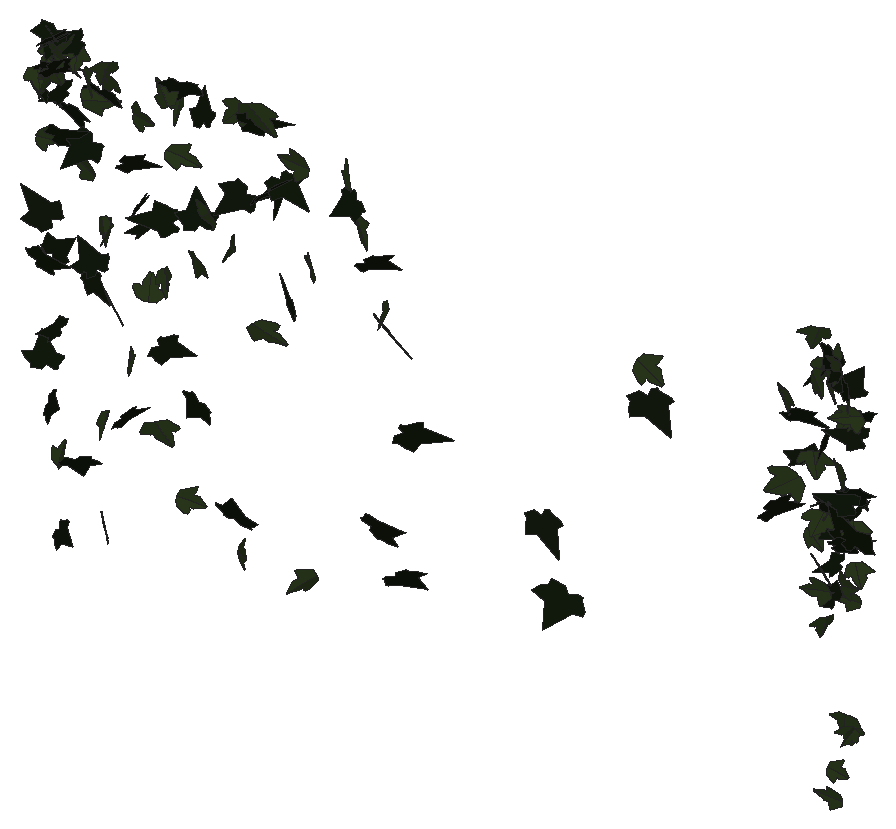
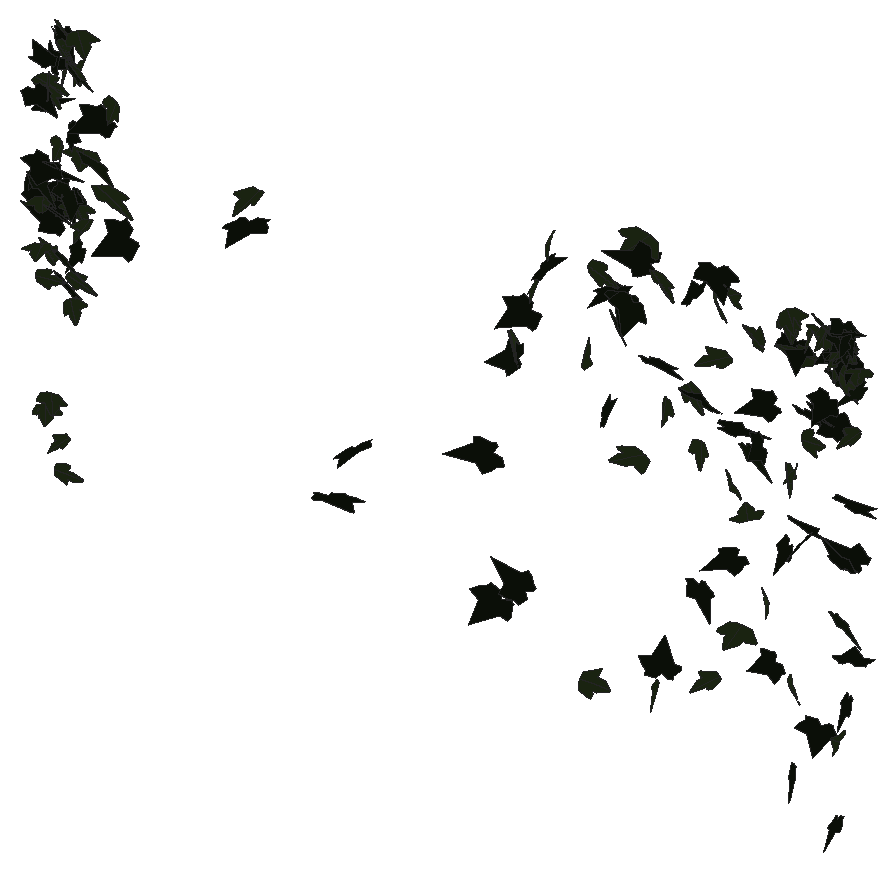
# SketchUp Ruby script. Lengths in inches.
U = 1.inch
M = Sketchup.active_model
def pt(a) = Geom::Point3d.new(a.map { |v| v * U })
def face(e, loops, mat)
  f = e.add_face(loops[0].map { |a| pt(a) })
  loops[1..].each { |l| e.add_face(l.map { |a| pt(a) }).erase! }
  f.material = f.back_material = mat if mat
  f
end
# faces: each face lists its corners as indices into pts; further lists are holes
def faces(e, pts, list, mat = nil) = list.each { |f| face(e, (f[0].is_a?(Array) ? f : [f]).map { |l| l.map { |i| pts[i] } }, mat) }
# xy, xz, yz: faces in a plane at the given z, y or x. An outline is a flat list of corners, or four numbers for a rectangle; further outlines are holes
def ring(l) = l.size == 4 ? [[l[0], l[1]], [l[2], l[1]], [l[2], l[3]], [l[0], l[3]]] : l.each_slice(2).to_a
def flat(e, list, mat, &to3) = list.each { |f| face(e, (f[0].is_a?(Array) ? f : [f]).map { |l| ring(l).map { |u, v| to3.(u, v) } }, mat) }
def xy(e, z, list, mat = nil) = flat(e, list, mat) { |x, y| [x, y, z] }
def xz(e, y, list, mat = nil) = flat(e, list, mat) { |x, z| [x, y, z] }
def yz(e, x, list, mat = nil) = flat(e, list, mat) { |y, z| [x, y, z] }
def lines(e, pts, list) = list.each { |a, b| e.add_line(pt(pts[a]), pt(pts[b])) }
# prism: a flat outline (further loops are holes) pulled along v
def prism(e, loops, v, mat = nil)
  f = face(e, loops, mat); d = Geom::Vector3d.new(v.map { |x| x * U })
  f.pushpull(f.normal.samedirection?(d) ? d.length : -d.length)
end
def box(e, o, s, mat = nil) = prism(e, [[o, [o[0] + s[0], o[1], o[2]], [o[0] + s[0], o[1] + s[1], o[2]], [o[0], o[1] + s[1], o[2]]]], [0, 0, s[2]], mat)
def at(x, y, z, deg = 0) = Geom::Transformation.translation(pt([x, y, z])) * Geom::Transformation.rotation(ORIGIN, Z_AXIS, deg.degrees)
def axes(o, x, y, z) = Geom::Transformation.new([*x, 0, *y, 0, *z, 0, *pt(o).to_a, 1])
def part(name) = M.definitions.add(name)
# library, detail: a bought-in or finely detailed component or shape, given as its bounding box
def library(name, o, s) = part(name).tap { |d| box(d.entities, o, s) }
def detail(e, o, s) = box(e.add_group.entities, o, s)
def put(e, d, t, mat = nil) = e.add_instance(d, t).tap { |i| i.material = mat if mat }
def group(e, t, mat = nil) = e.add_group.tap { |g| g.transformation = t; g.material = mat if mat }.entities
root = M.entities
M.materials.add("1026 AP 7946 SUNNY SIDE UP").color = [254, 231, 186]
M.materials.add("efeu1").color = [18, 25, 13]
M.materials.add("efeu2").color = [43, 57, 29]
c1 = part("ivyleaf_9")
p = [[1.54,2.16,1.25],[1.36,2.04,1.19],[-0.21,0.99,0.68],[-0.71,1.11,0.82],[-0.85,0.86,0.67],[-0.8,0.17,0.21],
  [-0.9,-0.01,0.1],[-0.67,-0.16,-0.02],[-0.08,-0.08,-0.05],[-0.03,-0.6,-0.4],[0.65,-0.88,-0.66],[0.83,-0.6,-0.49],
  [1.29,-0.42,-0.43],[1.8125,-0.07,-0.26],[1.21,0.44,0.15]]
faces(c1.entities,p,[[0,1,2,3,4,5,6,7,8,9,10,11,12,13,14]],"efeu1")
c2 = part("ivyleaf_10")
p = [[0,0.5,-0.03],[-0.0625,2.02,-0.43],[-0.19,2.01,-0.46],[-0.54,1.05,-0.29],[-0.52,0.625,-0.18],[-0.83,0.76,-0.28],
  [-1.16,0.64,-0.33],[-1.15,0.33,-0.24],[-0.77,-0.39,0.02],[-0.3,-0.51,0.16],[0.04,-0.48,0.23],[-0.02,2.01,-0.4375],
  [-0.06,2.01,-0.43],[0.04,-0.49,0.23],[0.67,-0.49,0.14],[1.38,0.36,-0.2],[1.375,0.51,-0.24],[0.81,0.65,-0.19],
  [0.62,0.59,-0.15],[0.6,1.09,-0.28],[0.5,1.23,-0.31]]
faces(c2.entities,p,[[0,1,2,3,4,5,6,7,8,9,10],[11,12,0,13,14,15,16,17,18,19,20]],"efeu2")
put(root,c1,axes([117.92,212.64,266.27],[0.34447,-0.10221,-0.11424],[-0.10357,0.11002,-0.23912],[0.21258,0.21922,0.06863]),"1026 AP 7946 SUNNY SIDE UP")
put(root,c1,axes([118.2,212.71,258.34],[-0.36248,-0.06396,0.109],[0.15543,0.04038,0.24641],[-0.11757,0.25057,-0.01029]),"1026 AP 7946 SUNNY SIDE UP")
put(root,c2,axes([118.03,212.6,266.67],[0.26881,0.19626,0.00102],[0.01701,-0.00958,-0.26778],[-0.30813,0.17069,-0.01389]),"1026 AP 7946 SUNNY SIDE UP")
put(root,c1,axes([118.48,212.51,262.68],[-0.44152,-0.06357,-0.11525],[-0.18136,0.00727,0.29498],[-0.08856,0.30203,-0.02951]),"1026 AP 7946 SUNNY SIDE UP")
put(root,c2,axes([118.14,212.62,264.84],[0.01266,0.11269,0.23888],[0.00793,0.23124,-0.11493],[-0.40441,0.00806,0.00522]),"1026 AP 7946 SUNNY SIDE UP")
put(root,c1,axes([118.29,212.72,257.18],[0.05293,-0.0259,-0.29049],[-0.3113,0.20067,-0.04218],[0.31802,0.20074,0.00706]),"1026 AP 7946 SUNNY SIDE UP")
put(root,c2,axes([118.32,212.88,267.27],[0.23133,0.15211,-0.15112],[-0.14124,-0.11794,-0.2182],[-0.30182,0.17178,-0.01372]),"1026 AP 7946 SUNNY SIDE UP")
put(root,c2,axes([118.28,212.85,266.58],[0.05975,-0.23156,0.20577],[0.06281,-0.19713,-0.24282],[0.4781,0.05484,0.00619]),"1026 AP 7946 SUNNY SIDE UP")
put(root,c1,axes([118.08,213.03,267.7],[0.29837,-0.17045,0.00968],[-0.01091,-0.02317,-0.26194],[0.2683,0.18862,-0.02141]),"1026 AP 7946 SUNNY SIDE UP")
put(root,c1,axes([118.13,213.09,261.29],[-0.13636,0.13153,0.21387],[0.22426,-0.15138,0.15988],[0.31349,0.16551,-0.02134]),"1026 AP 7946 SUNNY SIDE UP")
put(root,c1,axes([117.99,212.66,261.23],[0.09601,-0.03822,0.25968],[0.32127,-0.14806,-0.07492],[0.24033,0.2132,-0.00359]),"1026 AP 7946 SUNNY SIDE UP")
put(root,c1,axes([118.45,212.75,267.66],[0.02147,0.25653,0.0187],[-0.01192,0.01711,-0.2644],[-0.40404,0.01313,0.0088]),"1026 AP 7946 SUNNY SIDE UP")
put(root,c1,axes([118.33,212.92,267.79],[-0.23433,-0.21118,-0.0017],[0.03878,-0.01686,-0.26458],[0.32978,-0.14807,0.0299]),"1026 AP 7946 SUNNY SIDE UP")
put(root,c1,axes([118.49,212.61,267.84],[-0.0099,0.25599,-0.03036],[0.00018,-0.03093,-0.26398],[-0.40545,-0.00627,0.00062]),"1026 AP 7946 SUNNY SIDE UP")
put(root,c2,axes([118.34,212.91,267.35],[-0.08937,0.25025,-0.01074],[-0.00659,-0.01309,-0.26436],[-0.39389,-0.05656,0.00686]),"1026 AP 7946 SUNNY SIDE UP")
put(root,c1,axes([118.62,212.71,259.44],[-0.23134,0.21492,0.03365],[-0.04737,0.01742,-0.26778],[-0.33824,-0.14944,0.01449]),"1026 AP 7946 SUNNY SIDE UP")
put(root,c1,axes([118.47,212.64,267.02],[0.21167,0.214,-0.09142],[-0.05465,-0.08423,-0.26051],[-0.3609,0.13827,-0.01417]),"1026 AP 7946 SUNNY SIDE UP")
put(root,c2,axes([118.73,212.51,267.39],[0.03224,-0.0236,-0.2805],[-0.31872,0.18164,-0.0309],[0.28795,0.20369,-0.0028]),"1026 AP 7946 SUNNY SIDE UP")
put(root,c2,axes([118.45,212.69,266.86],[-0.20915,-0.21356,-0.11347],[0.13001,0.07607,-0.2572],[0.35384,-0.15418,0.02743]),"1026 AP 7946 SUNNY SIDE UP")
put(root,c1,axes([118.26,212.88,267.28],[0.2693,-0.19309,-0.00503],[0.06195,0.03988,-0.25934],[0.29728,0.1666,0.0586]),"1026 AP 7946 SUNNY SIDE UP")
put(root,c1,axes([118.59,212.78,253.63],[0.098,-0.10726,-0.25094],[-0.24061,0.18949,-0.1255],[0.34134,0.16436,-0.01642]),"1026 AP 7946 SUNNY SIDE UP")
put(root,c1,axes([118.83,212.6875,266.38],[-0.2985,0.17637,-0.00799],[-0.01055,-0.02004,-0.26632],[-0.27746,-0.18898,0.01871]),"1026 AP 7946 SUNNY SIDE UP")
put(root,c2,axes([118.7,212.9,267.56],[-0.05796,-0.25516,0.02452],[0.01005,-0.02641,-0.26555],[0.40305,-0.03603,0.01015]),"1026 AP 7946 SUNNY SIDE UP")
put(root,c2,axes([118.71,212.54,255.78],[0.0181,0.14274,-0.22667],[0.0407,0.21936,0.14874],[0.41145,-0.02798,-0.00474]),"1026 AP 7946 SUNNY SIDE UP")
put(root,c1,axes([118.61,212.36,267.09],[0.2386,0.18431,0.18808],[0.20633,0.12653,-0.24461],[-0.35056,0.19992,-0.01596]),"1026 AP 7946 SUNNY SIDE UP")
put(root,c1,axes([118.5,212.73,264.95],[0.3529,0.092,-0.10758],[0.10626,0.10225,0.24182],[0.19201,-0.22567,0.06389]),"1026 AP 7946 SUNNY SIDE UP")
put(root,c1,axes([118.74,212.95,265.76],[0.38897,0.00534,-0.08902],[-0.13488,-0.021,-0.25435],[-0.0188,0.2612,-0.01709]),"1026 AP 7946 SUNNY SIDE UP")
put(root,c2,axes([118.83,212.89,267.68],[-0.09661,-0.19451,-0.1674],[0.11101,0.14627,-0.20845],[0.3816,-0.0918,0.01826]),"1026 AP 7946 SUNNY SIDE UP")
put(root,c1,axes([119.16,212.8125,267.86],[-0.35541,0.12461,-0.0421],[0.04217,-0.03722,-0.26536],[-0.2022,-0.22679,0.01866]),"1026 AP 7946 SUNNY SIDE UP")
put(root,c2,axes([119.04,212.82,267.55],[0.39368,-0.02427,0.06501],[0.09332,-0.03811,-0.25736],[0.05134,0.2554,-0.03068]),"1026 AP 7946 SUNNY SIDE UP")
put(root,c2,axes([119.53,212.78,264.26],[-0.1002,0.04016,-0.26145],[-0.30999,0.16041,0.07802],[0.25966,0.207,-0.00775]),"1026 AP 7946 SUNNY SIDE UP")
put(root,c1,axes([119.31,212.53,255.99],[0.25437,0.20472,-0.04995],[-0.03412,-0.04608,-0.26881],[-0.32947,0.16283,-0.01073]),"1026 AP 7946 SUNNY SIDE UP")
put(root,c1,axes([119.54,212.8,265.08],[-0.48829,-0.0222,-0.05],[0.07902,-0.02729,-0.31935],[0.02773,-0.3131,0.02953]),"1026 AP 7946 SUNNY SIDE UP")
put(root,c1,axes([119.84,212.66,261.65],[-0.41695,0.00863,-0.09009],[-0.13564,0.02814,0.27236],[0.02669,0.27781,-0.02315]),"1026 AP 7946 SUNNY SIDE UP")
put(root,c2,axes([119.64,212.53,267.17],[-0.16324,0.25393,0.00579],[-0.02087,-0.00091,-0.28232],[-0.39878,-0.1039,0.0124]),"1026 AP 7946 SUNNY SIDE UP")
put(root,c1,axes([119.66,212.65,261.36],[0.1944,-0.19744,-0.15862],[-0.12045,0.13234,-0.23917],[0.37368,0.14538,0.00543]),"1026 AP 7946 SUNNY SIDE UP")
put(root,c2,axes([119.78,213.09,257.17],[0.23626,-0.16688,0.17491],[0.15028,-0.14282,-0.23129],[0.34401,0.177,-0.01909]),"1026 AP 7946 SUNNY SIDE UP")
put(root,c1,axes([120.02,212.61,266.82],[0.32573,0.06849,-0.16469],[-0.22442,-0.07618,-0.22405],[-0.15726,0.25058,-0.02139]),"1026 AP 7946 SUNNY SIDE UP")
put(root,c2,axes([119.72,212.5625,266.5],[0.10202,-0.01231,-0.28526],[0.4343,0.02581,0.06566],[0.03515,-0.28316,0.01672]),"1026 AP 7946 SUNNY SIDE UP")
put(root,c1,axes([120.13,212.6,254.47],[0.19015,-0.08255,-0.23249],[-0.32342,0.09406,-0.14875],[0.19402,0.23769,-0.0201]),"1026 AP 7946 SUNNY SIDE UP")
put(root,c2,axes([120.21,212.66,267.58],[-0.16601,-0.24648,0.0507],[-0.0152,-0.05088,-0.2763],[0.39536,-0.10545,0.01067]),"1026 AP 7946 SUNNY SIDE UP")
put(root,c2,axes([120.13,212.59,263.07],[-0.03713,0.25729,-0.06699],[0.00702,-0.06635,-0.26655],[-0.41779,-0.02398,0.00147]),"1026 AP 7946 SUNNY SIDE UP")
put(root,c2,axes([120.33,212.5625,267.33],[-0.36104,0.08554,0.10624],[-0.16165,0.01723,-0.25162],[-0.13418,-0.25091,0.01729]),"1026 AP 7946 SUNNY SIDE UP")
put(root,c2,axes([120.34,212.54,263.01],[0.08925,-0.27384,-0.15193],[-0.02542,0.14553,-0.28698],[0.48724,0.05775,0.01286]),"1026 AP 7946 SUNNY SIDE UP")
put(root,c1,axes([120.27,212.66,260.9],[0.32555,-0.11074,-0.15892],[-0.23022,0.05078,-0.24068],[0.18888,0.25276,-0.01945]),"1026 AP 7946 SUNNY SIDE UP")
put(root,c1,axes([120.59,212.8,257.52],[-0.06695,0.16434,-0.23012],[-0.09669,0.21574,0.17612],[0.42641,0.07472,0.0038]),"1026 AP 7946 SUNNY SIDE UP")
put(root,c2,axes([120.85,212.77,259.09],[0.1432,-0.09556,0.25591],[-0.24416,0.19486,0.13672],[-0.34088,-0.17972,0.00958]),"1026 AP 7946 SUNNY SIDE UP")
put(root,c1,axes([120.69,212.8,264.89],[0.24543,0.11893,0.19398],[0.25639,0.09438,-0.20083],[-0.23721,0.22507,-0.01637]),"1026 AP 7946 SUNNY SIDE UP")
put(root,c1,axes([120.96,212.85,263.61],[0.05266,0.14761,0.2346],[0.11264,0.21564,-0.15415],[-0.41044,0.07811,-0.0122]),"1026 AP 7946 SUNNY SIDE UP")
put(root,c1,axes([121.41,212.79,263.36],[-0.2316,0.232,0.00463],[-0.02415,-0.00599,-0.28265],[-0.36403,-0.1472,0.0158]),"1026 AP 7946 SUNNY SIDE UP")
put(root,c2,axes([121.13,212.68,266.47],[-0.09464,0.03818,0.27329],[0.40331,-0.0699,0.06997],[0.12109,0.26267,-0.01943]),"1026 AP 7946 SUNNY SIDE UP")
put(root,c2,axes([121.4375,212.78,261.375],[0.25705,0.20502,-0.08424],[0.04965,0.08044,0.26945],[0.34419,-0.16472,0.02404]),"1026 AP 7946 SUNNY SIDE UP")
put(root,c1,axes([122.14,212.77,263.73],[-0.31735,0.01216,0.19622],[-0.29978,-0.02326,-0.2068],[0.01126,-0.27648,0.02439]),"1026 AP 7946 SUNNY SIDE UP")
put(root,c2,axes([121.92,212.57,257.87],[-0.36095,-0.15018,-0.12502],[0.18721,0.03665,-0.28051],[0.23795,-0.25666,0.03105]),"1026 AP 7946 SUNNY SIDE UP")
put(root,c1,axes([121.88,212.74,260.08],[0.06867,0.01812,-0.29073],[-0.01866,0.28552,0.01866],[0.44443,0.00919,0.04571]),"1026 AP 7946 SUNNY SIDE UP")
put(root,c2,axes([122.23,212.51,267.35],[0.30286,-0.02582,0.19911],[-0.28409,0.07907,0.19669],[-0.11592,-0.26126,0.03817]),"1026 AP 7946 SUNNY SIDE UP")
put(root,c2,axes([121.93,212.78,262.15],[0.26319,-0.10413,0.19726],[0.24102,-0.11645,-0.20333],[0.24481,0.2266,-0.01189]),"1026 AP 7946 SUNNY SIDE UP")
put(root,c2,axes([122.3125,212.9,267.23],[0.2864,-0.18115,0.15014],[0.14405,-0.11565,-0.26487],[0.33711,0.20333,-0.01437]),"1026 AP 7946 SUNNY SIDE UP")
put(root,c2,axes([122.23,212.82,265.71],[0.11509,0.11581,0.24927],[0.23738,0.18872,-0.13937],[-0.34754,0.16725,-0.01265]),"1026 AP 7946 SUNNY SIDE UP")
put(root,c1,axes([122.62,212.55,267.97],[0.23206,0.17209,-0.1592],[-0.14344,-0.1264,-0.23403],[-0.33531,0.17317,-0.01006]),"1026 AP 7946 SUNNY SIDE UP")
put(root,c1,axes([123.02,212.78,258.84],[0.22682,-0.00329,-0.26037],[-0.39301,-0.04503,-0.14663],[-0.05896,0.28748,-0.02423]),"1026 AP 7946 SUNNY SIDE UP")
put(root,c2,axes([122.99,212.79,262.88],[-0.34003,0.14679,0.10208],[-0.14449,0.03915,-0.26839],[-0.23721,-0.23428,0.01716]),"1026 AP 7946 SUNNY SIDE UP")
put(root,c2,axes([122.8,212.5,256.125],[0.04278,0.13555,0.25],[0.09288,0.23466,-0.14093],[-0.42601,0.06477,-0.00562]),"1026 AP 7946 SUNNY SIDE UP")
put(root,c1,axes([123.14,212.7,264.09],[-0.44397,0.07696,-0.00406],[0.00274,0.02299,0.30072],[0.12118,0.28145,-0.02167]),"1026 AP 7946 SUNNY SIDE UP")
put(root,c2,axes([123.34,212.74,264.36],[-0.27865,0.07859,0.21199],[-0.32347,0.03377,-0.19603],[-0.12197,-0.26912,0.03557]),"1026 AP 7946 SUNNY SIDE UP")
put(root,c1,axes([123.24,212.72,267.0625],[-0.14769,-0.14091,0.23108],[0.19785,0.18666,0.17555],[-0.36775,0.15701,0.00164]),"1026 AP 7946 SUNNY SIDE UP")
put(root,c2,axes([124.07,213.09,267.51],[0.35062,-0.15638,-0.13321],[-0.17487,0.06493,-0.28002],[0.26581,0.24899,-0.00851]),"1026 AP 7946 SUNNY SIDE UP")
put(root,c2,axes([124.08,212.76,263.71],[0.0108,-0.19312,-0.21778],[-0.00123,0.21035,-0.19779],[0.44896,0.00522,0.0047]),"1026 AP 7946 SUNNY SIDE UP")
put(root,c1,axes([124.22,213.15,265.09],[-0.43848,-0.05221,0.00728],[-0.00338,-0.02835,-0.29107],[0.08283,-0.27752,0.02667]),"1026 AP 7946 SUNNY SIDE UP")
put(root,c1,axes([124.23,212.76,255.96],[0.41984,-0.09545,0.08544],[-0.10813,0.05451,0.29111],[-0.16753,-0.27439,0.02625]),"1026 AP 7946 SUNNY SIDE UP")
put(root,c2,axes([124.66,212.46,255.2],[-0.11348,0.17055,0.2265],[-0.18556,0.18583,-0.18817],[-0.3949,-0.13633,0.02333]),"1026 AP 7946 SUNNY SIDE UP")
put(root,c1,axes([124.72,212.68,267.5],[0.17484,0.02898,0.28489],[0.43204,0.03302,-0.11726],[-0.06531,0.29606,-0.01304]),"1026 AP 7946 SUNNY SIDE UP")
put(root,c2,axes([124.98,212.56,268.05],[-0.45132,0.0032,-0.18636],[0.28249,-0.03535,-0.29448],[-0.03387,-0.33744,0.02709]),"1026 AP 7946 SUNNY SIDE UP")
put(root,c2,axes([125.12,212.64,261.79],[-0.25215,-0.04244,-0.24375],[0.37214,0.02027,-0.16904],[0.06404,-0.28491,0.02257]),"1026 AP 7946 SUNNY SIDE UP")
put(root,c1,axes([125.5,212.36,265.9],[0.11817,0.29069,0.10689],[0.06,0.09551,-0.30849],[-0.48073,0.08337,-0.01223]),"1026 AP 7946 SUNNY SIDE UP")
put(root,c1,axes([125.4,213.14,265.73],[-0.22754,0.00424,-0.25662],[0.35992,-0.11152,-0.13959],[-0.15474,-0.26564,0.05267]),"1026 AP 7946 SUNNY SIDE UP")
put(root,c1,axes([125.67,212.35,266.04],[0.10429,0.2936,0.10669],[0.0523,0.09688,-0.30933],[-0.48587,0.07345,-0.0104]),"1026 AP 7946 SUNNY SIDE UP")
put(root,c2,axes([126.32,212.8,266.79],[0.07856,-0.05605,-0.30452],[-0.38815,0.16309,-0.07397],[0.26957,0.25117,-0.01776]),"1026 AP 7946 SUNNY SIDE UP")
put(root,c1,axes([126.15,212.68,262.6],[-0.01122,-0.18991,0.24222],[0.01015,0.23611,0.19715],[-0.47644,0.0095,-0.0015]),"1026 AP 7946 SUNNY SIDE UP")
put(root,c1,axes([125.87,212.57,266.3125],[0.06313,-0.19406,-0.22485],[0.02667,0.2204,-0.19838],[0.45716,0.01394,0.04262]),"1026 AP 7946 SUNNY SIDE UP")
put(root,c2,axes([126.5,212.93,254.94],[-0.04741,-0.14957,0.27445],[-0.07338,-0.26317,-0.15869],[0.47595,-0.05547,0.00287]),"1026 AP 7946 SUNNY SIDE UP")
put(root,c2,axes([126.78,212.66,263.95],[-0.28438,0.22785,0.04143],[0.05484,-0.02195,0.29923],[0.3593,0.18369,-0.01288]),"1026 AP 7946 SUNNY SIDE UP")
put(root,c2,axes([127.95,212.66,266.9],[-0.06458,0.18128,-0.24099],[-0.09968,0.22636,0.19266],[0.45585,0.07518,0.00799]),"1026 AP 7946 SUNNY SIDE UP")
put(root,c1,axes([127.95,212.9,266.32],[0.05792,-0.14147,-0.26744],[0.17038,-0.23608,0.14745],[-0.43133,-0.11225,0.02233]),"1026 AP 7946 SUNNY SIDE UP")
put(root,c2,axes([128.27,212.75,265.75],[-0.12906,0.28661,0.02041],[-0.02376,0.01458,-0.30685],[-0.45094,-0.08279,0.01032]),"1026 AP 7946 SUNNY SIDE UP")
put(root,c1,axes([128.52,212.73,264.82],[0.30752,0.17525,0.15376],[0.18879,0.0879,-0.2697],[-0.30763,0.22913,-0.01181]),"1026 AP 7946 SUNNY SIDE UP")
put(root,c1,axes([128.4,213.1,257],[0.42295,-0.00469,-0.16959],[0.25554,0.05834,0.27223],[0.0417,-0.3099,0.05194]),"1026 AP 7946 SUNNY SIDE UP")
put(root,c2,axes([129.21,212.5625,263.71],[0.15623,-0.29238,-0.12307],[-0.05999,0.11145,-0.31747],[0.49201,0.10643,0.00037]),"1026 AP 7946 SUNNY SIDE UP")
put(root,c1,axes([128.97,212.68,263.26],[0.35561,-0.20059,0.08339],[0.07568,-0.06919,-0.3112],[0.33228,0.23043,-0.01836]),"1026 AP 7946 SUNNY SIDE UP")
put(root,c1,axes([129.51,212.68,256.14],[0.34261,0.2073,0.10085],[0.13184,0.0519,-0.30889],[-0.33467,0.23267,-0.01844]),"1026 AP 7946 SUNNY SIDE UP")
put(root,c1,axes([129.72,212.75,260.3125],[0.13183,0.10607,-0.29413],[0.12237,0.27947,0.13187],[0.46394,-0.10385,0.0488]),"1026 AP 7946 SUNNY SIDE UP")
put(root,c1,axes([133.8125,213.1,259.17],[0.05535,-0.31108,-0.12549],[-0.02744,0.11883,-0.32179],[0.52357,0.03911,-0.0036]),"1026 AP 7946 SUNNY SIDE UP")
put(root,c1,axes([134.77,212.88,257.36],[-0.42187,-0.20535,-0.00502],[0.03084,-0.01955,-0.34703],[0.32148,-0.26761,0.02671]),"1026 AP 7946 SUNNY SIDE UP")
put(root,c2,axes([137.41,212.67,265.01],[0.07647,0.27653,0.20521],[0.06973,0.19277,-0.28799],[-0.52987,0.06527,-0.00828]),"1026 AP 7946 SUNNY SIDE UP")
put(root,c1,axes([137.58,212.67,264.14],[-0.03895,-0.25653,-0.2365],[0.02602,0.22754,-0.26414],[0.53915,-0.02951,-0.00433]),"1026 AP 7946 SUNNY SIDE UP")
put(root,c1,axes([141.48,212.63,262.3],[0.21157,0.20608,0.26696],[0.26385,0.19723,-0.25132],[-0.44712,0.2139,-0.02198]),"1026 AP 7946 SUNNY SIDE UP")
put(root,c2,axes([142.18,212.65,263.41],[0.42883,-0.09739,-0.21899],[-0.33233,0.03504,-0.29644],[0.15541,0.34366,-0.02964]),"1026 AP 7946 SUNNY SIDE UP")
put(root,c2,axes([142,212.57,265.91],[-0.32749,0.18764,-0.03223],[0.00813,-0.04236,-0.28762],[-0.29929,-0.20647,0.02746]),"1026 AP 7946 SUNNY SIDE UP")
put(root,c1,axes([142.62,212.68,264.2],[-0.12241,0.24306,0.08538],[-0.16021,0.04882,-0.24998],[-0.3699,-0.10158,0.08002]),"1026 AP 7946 SUNNY SIDE UP")
put(root,c1,axes([142.3,212.56,265.4],[0.37782,0.09033,0.11088],[0.16035,0.03308,-0.26421],[-0.15108,0.26099,-0.00315]),"1026 AP 7946 SUNNY SIDE UP")
put(root,c2,axes([142.8,212.94,267.78],[-0.27491,-0.18708,0.05127],[-0.03155,-0.05062,-0.26331],[0.30319,-0.1749,0.01909]),"1026 AP 7946 SUNNY SIDE UP")
put(root,c1,axes([143,212.99,266.86],[-0.2925,0.12941,-0.11953],[0.12689,-0.08742,-0.23277],[-0.24292,-0.20148,0.02233]),"1026 AP 7946 SUNNY SIDE UP")
put(root,c2,axes([143.19,212.66,260.56],[0.14753,-0.05959,-0.23649],[-0.34389,0.07282,-0.1113],[0.14292,0.23673,-0.02369]),"1026 AP 7946 SUNNY SIDE UP")
put(root,c2,axes([142.85,212.69,264.29],[0.3659,0.12996,0.04262],[0.03874,0.03895,-0.27344],[-0.21058,0.23299,0.02376]),"1026 AP 7946 SUNNY SIDE UP")
put(root,c2,axes([142.95,212.98,266.84],[0.34627,-0.13159,0.02014],[0.01144,-0.02728,-0.26367],[0.20905,0.21946,-0.01894]),"1026 AP 7946 SUNNY SIDE UP")
put(root,c2,axes([142.91,212.54,262.18],[0.04693,0.24269,0.11297],[0.02371,0.10724,-0.25127],[-0.4172,0.03339,-0.00157]),"1026 AP 7946 SUNNY SIDE UP")
put(root,c2,axes([143.0625,212.52,266.71],[-0.08256,0.27717,0.0751],[-0.04715,0.06679,-0.28973],[-0.44755,-0.05817,0.01667]),"1026 AP 7946 SUNNY SIDE UP")
put(root,c1,axes([143.1875,212.78,263.12],[0.08549,0.25106,0.03794],[-0.03133,0.04033,-0.26285],[-0.39743,0.05082,0.02888]),"1026 AP 7946 SUNNY SIDE UP")
put(root,c2,axes([143.12,212.66,262.66],[0.38905,0.06754,-0.06265],[-0.08337,-0.03734,-0.26351],[-0.11656,0.25213,-0.02063]),"1026 AP 7946 SUNNY SIDE UP")
put(root,c1,axes([143.07,212.55,261.39],[0.30507,-0.08976,-0.12388],[-0.17546,0.04386,-0.21988],[0.15678,0.22373,-0.00502]),"1026 AP 7946 SUNNY SIDE UP")
put(root,c1,axes([143.26,212.7,263.02],[0.22642,0.01006,-0.21022],[-0.32083,-0.00687,-0.14868],[-0.01794,0.2497,0.00584]),"1026 AP 7946 SUNNY SIDE UP")
put(root,c1,axes([143.14,212.86,264.87],[-0.10861,0.04231,-0.24464],[0.26966,-0.16544,-0.08264],[-0.26723,-0.18414,0.01604]),"1026 AP 7946 SUNNY SIDE UP")
put(root,c1,axes([143.45,212.75,260.375],[-0.09454,0.12867,0.21081],[-0.16101,0.17662,-0.1449],[-0.34323,-0.1183,0.00991]),"1026 AP 7946 SUNNY SIDE UP")
put(root,c1,axes([143.44,212.95,261.29],[-0.28532,0.15919,0.00492],[-0.02491,-0.01221,-0.24792],[-0.24914,-0.18108,0.01916]),"1026 AP 7946 SUNNY SIDE UP")
put(root,c2,axes([143.22,212.77,262.68],[0.12588,-0.19729,0.13444],[-0.06475,0.12525,0.21993],[-0.36725,-0.0897,0.00731]),"1026 AP 7946 SUNNY SIDE UP")
put(root,c2,axes([143.28,212.625,259.77],[-0.10776,-0.2426,0.01401],[0.00579,-0.01659,-0.25967],[0.38215,-0.06816,0.00788]),"1026 AP 7946 SUNNY SIDE UP")
put(root,c1,axes([143.55,212.58,267.48],[0.19227,-0.02065,-0.26848],[-0.41073,-0.00166,-0.12619],[0.01143,0.28776,-0.01831]),"1026 AP 7946 SUNNY SIDE UP")
put(root,c2,axes([143.62,212.6,267.0625],[0.14578,-0.09032,-0.23336],[-0.23043,0.17238,-0.13189],[0.30556,0.17309,0.01187]),"1026 AP 7946 SUNNY SIDE UP")
put(root,c2,axes([143.69,212.56,254.79],[0.01412,-0.00996,-0.23013],[-0.33823,0.06048,-0.01133],[0.09573,0.21517,-0.0061]),"1026 AP 7946 SUNNY SIDE UP")
put(root,c2,axes([143.51,212.54,266.59],[-0.21296,0.21999,0.09978],[-0.09023,0.07689,-0.26556],[-0.36622,-0.14687,0.0074]),"1026 AP 7946 SUNNY SIDE UP")
put(root,c2,axes([143.76,212.51,267.45],[0.01803,0.06092,0.27026],[-0.38899,0.10533,-0.01347],[-0.16604,-0.24016,0.06089]),"1026 AP 7946 SUNNY SIDE UP")
put(root,c1,axes([143.73,212.9,262.46],[-0.38049,0.07611,0.01374],[-0.03388,-0.02583,-0.25951],[-0.11656,-0.24094,0.0306]),"1026 AP 7946 SUNNY SIDE UP")
put(root,c1,axes([143.81,212.53,267.24],[-0.1603,0.00786,-0.27583],[-0.3973,0.09242,0.10243],[0.14003,0.27123,-0.02514]),"1026 AP 7946 SUNNY SIDE UP")
put(root,c2,axes([143.64,212.71,264.25],[-0.26516,0.20139,-0.0655],[0.03136,-0.06727,-0.26955],[-0.33113,-0.16764,0.02692]),"1026 AP 7946 SUNNY SIDE UP")
put(root,c2,axes([143.78,212.86,257.02],[-0.34469,-0.03621,0.03081],[-0.03711,-0.03959,-0.22628],[0.06407,-0.2177,0.03468]),"1026 AP 7946 SUNNY SIDE UP")
put(root,c2,axes([143.65,212.47,255.67],[0.03641,0.14043,0.18617],[0.04505,0.17763,-0.14559],[-0.35604,0.03684,0.00062]),"1026 AP 7946 SUNNY SIDE UP")
put(root,c2,axes([143.99,212.92,260.44],[-0.00705,-0.01243,-0.22824],[-0.34853,0.00899,0.00415],[0.01376,0.22134,-0.01168]),"1026 AP 7946 SUNNY SIDE UP")
put(root,c1,axes([144.12,212.6,263.37],[-0.23248,0.06675,0.19398],[-0.29167,0.03986,-0.1647],[-0.11513,-0.23576,0.02554]),"1026 AP 7946 SUNNY SIDE UP")
put(root,c1,axes([143.93,212.6,266.49],[0.04946,-0.09218,0.27143],[-0.04103,0.26354,0.09954],[-0.43777,-0.03511,0.02134]),"1026 AP 7946 SUNNY SIDE UP")
put(root,c2,axes([143.9,212.91,256.69],[-0.24526,-0.15487,-0.00379],[0.02545,-0.01234,-0.22556],[0.24223,-0.15551,0.01986]),"1026 AP 7946 SUNNY SIDE UP")
put(root,c2,axes([144.03,212.66,266.01],[-0.16771,0.14504,0.19726],[-0.20597,0.13942,-0.18394],[-0.31537,-0.16819,0.01523]),"1026 AP 7946 SUNNY SIDE UP")
put(root,c2,axes([144.01,212.77,265.77],[0.3453,-0.07401,-0.09413],[-0.14802,0.00383,-0.23736],[0.10992,0.23766,-0.02396]),"1026 AP 7946 SUNNY SIDE UP")
put(root,c1,axes([143.67,212.66,262.04],[0.24394,0.17574,-0.12253],[0.10553,0.10043,0.24163],[0.31747,-0.16842,0.01383]),"1026 AP 7946 SUNNY SIDE UP")
put(root,c2,axes([144.19,212.67,265.93],[0.21641,-0.01961,-0.22858],[-0.35002,-0.0165,-0.14091],[-0.00589,0.26048,-0.0246]),"1026 AP 7946 SUNNY SIDE UP")
put(root,c2,axes([144.01,212.84,256.68],[0.02251,0.13985,-0.1737],[-0.12447,-0.15508,-0.13968],[-0.32221,0.06967,0.04182]),"1026 AP 7946 SUNNY SIDE UP")
put(root,c1,axes([144.12,213.03,265.8],[-0.01878,0.17269,-0.17487],[-0.06119,-0.17008,-0.17543],[-0.3769,0.01901,0.03719]),"1026 AP 7946 SUNNY SIDE UP")
put(root,c1,axes([143.89,212.76,266.54],[-0.25937,0.03676,0.19328],[0.28652,-0.04384,0.17383],[0.0899,0.24578,0.00361]),"1026 AP 7946 SUNNY SIDE UP")
put(root,c1,axes([144.25,212.79,265.25],[-0.14264,-0.01308,0.24397],[-0.34312,-0.09493,-0.09204],[0.14641,-0.23523,0.02197]),"1026 AP 7946 SUNNY SIDE UP")
put(root,c1,axes([144.25,212.58,262.31],[0.27803,-0.10908,0.30911],[-0.35331,0.20214,0.21285],[-0.35792,-0.28427,0.03]),"1026 AP 7946 SUNNY SIDE UP")
put(root,c1,axes([143.97,212.72,263.62],[0.33364,0.16059,0.00113],[0.02186,-0.01807,-0.27324],[-0.25157,0.21141,-0.02225]),"1026 AP 7946 SUNNY SIDE UP")
put(root,c1,axes([144.26,212.83,263.18],[-0.18753,0.22762,-0.02343],[-0.0004,-0.02724,-0.26456],[-0.35989,-0.11857,0.01251]),"1026 AP 7946 SUNNY SIDE UP")
put(root,c2,axes([144.03,212.85,262.62],[0.21497,0.21509,-0.0243],[-0.02034,-0.02118,-0.26268],[-0.33984,0.13732,0.00035]),"1026 AP 7946 SUNNY SIDE UP")
put(root,c2,axes([143.99,212.99,261.35],[0.21522,0.20012,0.02545],[0.03654,0.01262,-0.24939],[-0.31473,0.13831,-0.01155]),"1026 AP 7946 SUNNY SIDE UP")
put(root,c2,axes([143.87,212.65,260.92],[-0.171,0.06662,0.2291],[0.33721,-0.06412,0.12767],[0.13828,0.23875,-0.02803]),"1026 AP 7946 SUNNY SIDE UP")
